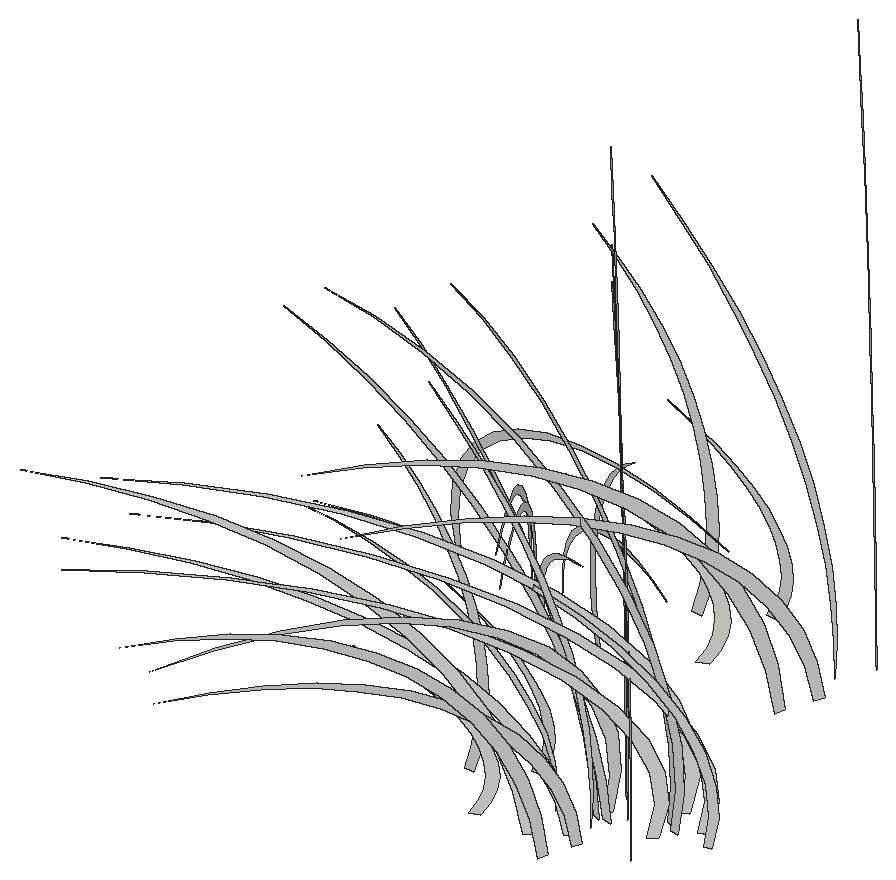
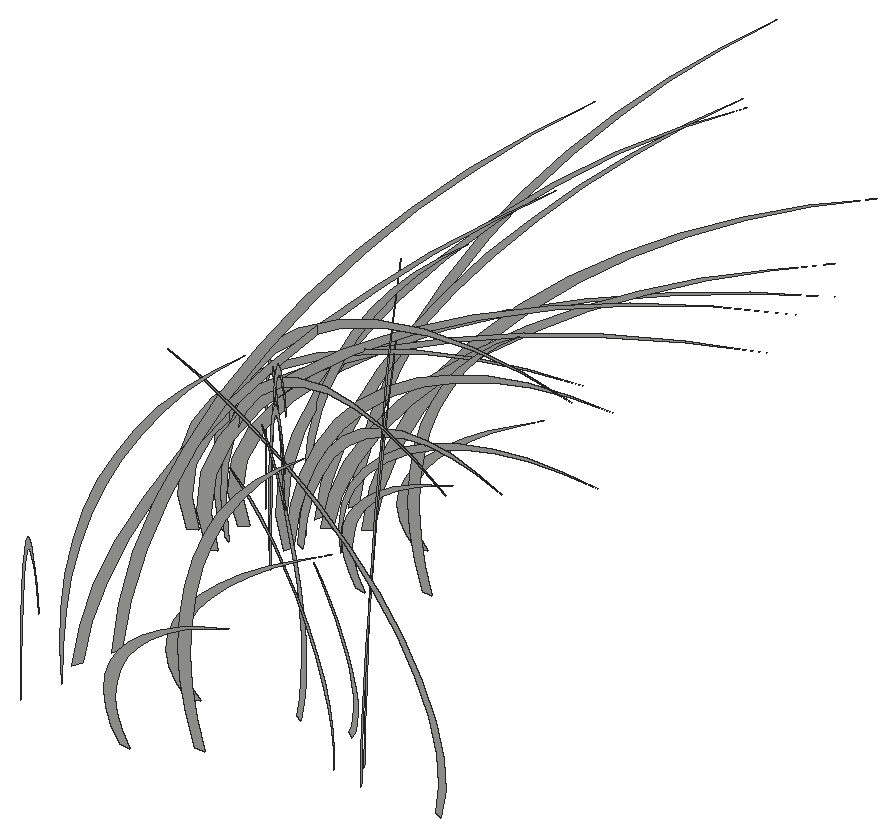
# SketchUp Ruby script. Lengths in inches.
U = 1.inch
M = Sketchup.active_model
def pt(a) = Geom::Point3d.new(a.map { |v| v * U })
def face(e, loops, mat)
  f = e.add_face(loops[0].map { |a| pt(a) })
  loops[1..].each { |l| e.add_face(l.map { |a| pt(a) }).erase! }
  f.material = f.back_material = mat if mat
  f
end
# faces: each face lists its corners as indices into pts; further lists are holes
def faces(e, pts, list, mat = nil) = list.each { |f| face(e, (f[0].is_a?(Array) ? f : [f]).map { |l| l.map { |i| pts[i] } }, mat) }
# xy, xz, yz: faces in a plane at the given z, y or x. An outline is a flat list of corners, or four numbers for a rectangle; further outlines are holes
def ring(l) = l.size == 4 ? [[l[0], l[1]], [l[2], l[1]], [l[2], l[3]], [l[0], l[3]]] : l.each_slice(2).to_a
def flat(e, list, mat, &to3) = list.each { |f| face(e, (f[0].is_a?(Array) ? f : [f]).map { |l| ring(l).map { |u, v| to3.(u, v) } }, mat) }
def xy(e, z, list, mat = nil) = flat(e, list, mat) { |x, y| [x, y, z] }
def xz(e, y, list, mat = nil) = flat(e, list, mat) { |x, z| [x, y, z] }
def yz(e, x, list, mat = nil) = flat(e, list, mat) { |y, z| [x, y, z] }
def lines(e, pts, list) = list.each { |a, b| e.add_line(pt(pts[a]), pt(pts[b])) }
# prism: a flat outline (further loops are holes) pulled along v
def prism(e, loops, v, mat = nil)
  f = face(e, loops, mat); d = Geom::Vector3d.new(v.map { |x| x * U })
  f.pushpull(f.normal.samedirection?(d) ? d.length : -d.length)
end
def box(e, o, s, mat = nil) = prism(e, [[o, [o[0] + s[0], o[1], o[2]], [o[0] + s[0], o[1] + s[1], o[2]], [o[0], o[1] + s[1], o[2]]]], [0, 0, s[2]], mat)
def at(x, y, z, deg = 0) = Geom::Transformation.translation(pt([x, y, z])) * Geom::Transformation.rotation(ORIGIN, Z_AXIS, deg.degrees)
def axes(o, x, y, z) = Geom::Transformation.new([*x, 0, *y, 0, *z, 0, *pt(o).to_a, 1])
def part(name) = M.definitions.add(name)
# library, detail: a bought-in or finely detailed component or shape, given as its bounding box
def library(name, o, s) = part(name).tap { |d| box(d.entities, o, s) }
def detail(e, o, s) = box(e.add_group.entities, o, s)
def put(e, d, t, mat = nil) = e.add_instance(d, t).tap { |i| i.material = mat if mat }
def group(e, t, mat = nil) = e.add_group.tap { |g| g.transformation = t; g.material = mat if mat }.entities
root = M.entities
g1 = group(root,at(18.37,764.86,-58.625))
p = [[3.01,-1.98,3.36],[2.46,-1.62,3.15],[1.96,-1.29,2.92],[1.52,-1,2.66],[1.15,-0.75,2.4],[0.83,-0.55,2.12],
  [0.59,-0.39,1.82],[0.41,-0.27,1.52],[0.3125,-0.21,1.22],[0.28,-0.1875,0.91],[0.33,-0.21,0.6],[0.44,-0.29,0.3],
  [0.63,-0.41,0],[0.39,-0.25,0],[0.18,-0.12,0.3],[0.05,-0.03,0.61],[0,0,0.93],[0.03,-0.02,1.24],
  [0.15,-0.1,1.55],[0.34,-0.22,1.85],[0.61,-0.4,2.15],[0.96,-0.63,2.43],[1.38,-0.91,2.69],[1.86,-1.23,2.94],
  [2.41,-1.58,3.16]]
faces(g1,p,[[0,1,2,3,4,5,6,7,8,9,10,11,12,13,14,15,16,17,18,19,20,21,22,23,24]])
g2 = group(root,at(25.21,756.14,-58.625))
p = [[-9.2,-6.42,9.74],[-10.59,-7.39,10],[-9.24,-6.45,9.69],[-7.94,-5.54,9.26],[-6.71,-4.68,8.71],[-5.54,-3.87,8.06],
  [-4.47,-3.12,7.3],[-3.49,-2.44,6.45],[-2.625,-1.83,5.52],[-1.88,-1.31,4.52],[-1.26,-0.88,3.45],[-0.78,-0.54,2.33],
  [-0.4375,-0.3,1.18],[-0.24,-0.17,0],[0,0,0],[-0.16,-0.11,1.21],[-0.48,-0.34,2.39],[-0.96,-0.67,3.53],
  [-1.58,-1.1,4.625],[-2.34,-1.63,5.65],[-3.23,-2.25,6.6],[-4.24,-2.96,7.45],[-5.36,-3.74,8.2],[-6.57,-4.58,8.84],
  [-7.85,-5.48,9.35]]
faces(g2,p,[[0,1,2,3,4,5,6,7,8,9,10,11,12,13,14,15,16,17,18,19,20,21,22,23,24]])
g3 = group(root,at(22.1,767.41,-58.625))
p = [[-4.36,0.43,9.78],[-3.5625,0.35,9.15],[-2.84,0.28,8.47],[-2.21,0.22,7.74],[-1.66,0.16,6.96],[-1.21,0.12,6.15],
  [-0.85,0.08,5.3],[-0.6,0.06,4.43],[-0.45,0.04,3.54],[-0.41,0.04,2.65],[-0.47,0.05,1.75],[-0.64,0.0625,0.87],
  [-0.91,0.09,0],[-0.5625,0.06,0],[-0.26,0.03,0.88],[-0.07,0.01,1.78],[0,0,2.6875],[-0.05,0,3.6],
  [-0.21,0.02,4.5],[-0.49,0.05,5.39],[-0.89,0.09,6.24],[-1.39,0.14,7.06],[-2,0.2,7.83],[-2.7,0.26,8.54],
  [-3.49,0.34,9.19]]
faces(g3,p,[[0,1,2,3,4,5,6,7,8,9,10,11,12,13,14,15,16,17,18,19,20,21,22,23,24]])
g4 = group(root,at(22.1,767.41,-58.625))
p = [[-4.36,0.43,9.78],[-3.5625,0.35,9.15],[-2.84,0.28,8.47],[-2.21,0.22,7.74],[-1.66,0.16,6.96],[-1.21,0.12,6.15],
  [-0.85,0.08,5.3],[-0.6,0.06,4.43],[-0.45,0.04,3.54],[-0.41,0.04,2.65],[-0.47,0.05,1.75],[-0.64,0.0625,0.87],
  [-0.91,0.09,0],[-0.5625,0.06,0],[-0.26,0.03,0.88],[-0.07,0.01,1.78],[0,0,2.6875],[-0.05,0,3.6],
  [-0.21,0.02,4.5],[-0.49,0.05,5.39],[-0.89,0.09,6.24],[-1.39,0.14,7.06],[-2,0.2,7.83],[-2.7,0.26,8.54],
  [-3.49,0.34,9.19]]
faces(g4,p,[[0,1,2,3,4,5,6,7,8,9,10,11,12,13,14,15,16,17,18,19,20,21,22,23,24]])
g5 = group(root,at(26.37,757.75,-58.625))
p = [[-10.97,2.33,9.03],[-12.625,2.68,9.27],[-11.02,2.34,8.98],[-9.47,2.01,8.58],[-8,1.7,8.08],[-6.61,1.41,7.47],
  [-5.33,1.13,6.77],[-4.16,0.88,5.98],[-3.13,0.67,5.12],[-2.24,0.48,4.1875],[-1.5,0.32,3.2],[-0.93,0.2,2.16],
  [-0.52,0.11,1.09],[-0.29,0.0625,0],[0,0,0],[-0.19,0.04,1.12],[-0.57,0.12,2.22],[-1.14,0.24,3.28],
  [-1.88,0.4,4.29],[-2.79,0.59,5.24],[-3.85,0.82,6.11],[-5.06,1.08,6.9],[-6.39,1.36,7.6],[-7.83,1.67,8.19],
  [-9.37,1.99,8.67]]
faces(g5,p,[[0,1,2,3,4,5,6,7,8,9,10,11,12,13,14,15,16,17,18,19,20,21,22,23,24]])
g6 = group(root,at(26.02,757.7,-58.625))
p = [[-9.9,5.27,7.86],[-11.4,6.06,8.07],[-9.95,5.29,7.82],[-8.55,4.55,7.47],[-7.22,3.84,7.03],[-5.97,3.17,6.5],
  [-4.81,2.56,5.89],[-3.76,2,5.21],[-2.83,1.5,4.45],[-2.02,1.08,3.64],[-1.36,0.72,2.78],[-0.84,0.45,1.88],
  [-0.47,0.25,0.95],[-0.26,0.14,0],[0,0,0],[-0.17,0.09,0.97],[-0.52,0.28,1.93],[-1.03,0.55,2.85],
  [-1.7,0.9,3.73],[-2.52,1.34,4.56],[-3.48,1.85,5.32],[-4.57,2.43,6.01],[-5.77,3.07,6.61],[-7.07,3.76,7.125],
  [-8.46,4.5,7.54]]
faces(g6,p,[[0,1,2,3,4,5,6,7,8,9,10,11,12,13,14,15,16,17,18,19,20,21,22,23,24]])
g7 = group(root,at(17.03,766.43,-58.625))
p = [[5.875,-8.62,6.21],[6.76,-9.92,6.375],[5.9,-8.66,6.18],[5.07,-7.44,5.9],[4.28,-6.28,5.56],[3.54,-5.19,5.14],
  [2.85,-4.1875,4.66],[2.23,-3.27,4.11],[1.68,-2.46,3.52],[1.2,-1.76,2.88],[0.81,-1.18,2.2],[0.5,-0.73,1.49],
  [0.28,-0.41,0.75],[0.15,-0.22,0],[0,0,0],[0.1,-0.15,0.77],[0.31,-0.45,1.52],[0.61,-0.9,2.25],
  [1.01,-1.48,2.95],[1.49,-2.19,3.6],[2.0625,-3.03,4.21],[2.71,-3.98,4.75],[3.42,-5.02,5.23],[4.2,-6.15,5.63],
  [5.02,-7.36,5.96]]
faces(g7,p,[[0,1,2,3,4,5,6,7,8,9,10,11,12,13,14,15,16,17,18,19,20,21,22,23,24]])
g8 = group(root,at(24.98,757.38,-58.625))
p = [[-9.02,0.88,5.34],[-7.8125,0.77,5.31],[-6.62,0.65,5.18],[-5.47,0.54,4.96],[-4.38,0.43,4.65],[-3.38,0.33,4.26],
  [-2.48,0.24,3.79],[-1.71,0.17,3.26],[-1.07,0.1,2.67],[-0.58,0.06,2.04],[-0.25,0.02,1.375],[-0.08,0.01,0.69],
  [-0.08,0.01,0],[0,0,0.7],[-0.11,0.01,1.41],[-0.4,0.04,2.09],[-0.86,0.08,2.75],[-1.5,0.15,3.35],
  [-2.28,0.22,3.9],[-3.2,0.3125,4.37],[-4.24,0.42,4.76],[-5.36,0.53,5.06],[-6.55,0.64,5.26],[-7.78,0.76,5.35]]
faces(g8,p,[[0,1,2,3,4,5,6,7,8,9,10,11,12,13,14,15,16,17,18,19,20,21,22,23]])
g9 = group(root,at(22.55,757.62,-58.625))
p = [[-3.86,0.38,8.65],[-3.15,0.31,8.1],[-2.51,0.25,7.5],[-1.95,0.19,6.85],[-1.47,0.14,6.16],[-1.07,0.1,5.44],
  [-0.75,0.07,4.6875],[-0.53,0.05,3.92],[-0.4,0.04,3.13],[-0.36,0.04,2.34],[-0.42,0.04,1.55],[-0.57,0.06,0.77],
  [-0.81,0.08,0],[-0.5,0.05,0],[-0.23,0.02,0.78],[-0.0625,0.01,1.57],[0,0,2.38],[-0.04,0,3.1875],
  [-0.1875,0.02,3.99],[-0.4375,0.04,4.77],[-0.79,0.08,5.52],[-1.23,0.12,6.25],[-1.77,0.17,6.93],[-2.39,0.23,7.5625],
  [-3.09,0.3,8.14]]
faces(g9,p,[[0,1,2,3,4,5,6,7,8,9,10,11,12,13,14,15,16,17,18,19,20,21,22,23,24]])
g10 = group(root,at(22.55,757.62,-58.625))
p = [[-3.86,0.38,8.65],[-3.15,0.31,8.1],[-2.51,0.25,7.5],[-1.95,0.19,6.85],[-1.47,0.14,6.16],[-1.07,0.1,5.44],
  [-0.75,0.07,4.6875],[-0.53,0.05,3.92],[-0.4,0.04,3.13],[-0.36,0.04,2.34],[-0.42,0.04,1.55],[-0.57,0.06,0.77],
  [-0.81,0.08,0],[-0.5,0.05,0],[-0.23,0.02,0.78],[-0.0625,0.01,1.57],[0,0,2.38],[-0.04,0,3.1875],
  [-0.1875,0.02,3.99],[-0.4375,0.04,4.77],[-0.79,0.08,5.52],[-1.23,0.12,6.25],[-1.77,0.17,6.93],[-2.39,0.23,7.5625],
  [-3.09,0.3,8.14]]
faces(g10,p,[[0,1,2,3,4,5,6,7,8,9,10,11,12,13,14,15,16,17,18,19,20,21,22,23,24]])
g11 = group(root,at(26.0625,756.74,-58.625))
p = [[-9.2,-6.42,7.86],[-10.59,-7.39,8.07],[-9.24,-6.45,7.82],[-7.94,-5.54,7.47],[-6.71,-4.68,7.03],[-5.54,-3.87,6.5],
  [-4.47,-3.12,5.89],[-3.49,-2.44,5.21],[-2.625,-1.83,4.45],[-1.88,-1.31,3.64],[-1.26,-0.88,2.78],[-0.78,-0.54,1.88],
  [-0.4375,-0.3,0.95],[-0.24,-0.17,0],[0,0,0],[-0.16,-0.11,0.97],[-0.48,-0.34,1.93],[-0.96,-0.67,2.85],
  [-1.58,-1.1,3.73],[-2.34,-1.63,4.56],[-3.23,-2.25,5.32],[-4.24,-2.96,6.01],[-5.36,-3.74,6.61],[-6.57,-4.58,7.125],
  [-7.85,-5.48,7.54]]
faces(g11,p,[[0,1,2,3,4,5,6,7,8,9,10,11,12,13,14,15,16,17,18,19,20,21,22,23,24]])
g12 = group(root,at(14.26,766.49,-58.625))
p = [[0.46,-0.1875,0],[0.21,-0.08,0],[0,0,0.88],[0.08,-0.03,1.76],[0.45,-0.18,2.63],[1.1,-0.44,3.46],
  [2.01,-0.81,4.23],[3.16,-1.27,4.92],[4.51,-1.8125,5.51],[6.05,-2.43,6],[7.72,-3.1,6.36],[9.49,-3.81,6.59],
  [11.3125,-4.55,6.6875],[13.14,-5.28,6.64],[11.35,-4.5625,6.65],[9.57,-3.85,6.53],[7.85,-3.16,6.28],[6.23,-2.5,5.9],
  [4.74,-1.91,5.41],[3.43,-1.38,4.82],[2.31,-0.93,4.14],[1.43,-0.57,3.39],[0.79,-0.32,2.58],[0.41,-0.16,1.73],
  [0.3,-0.12,0.86]]
faces(g12,p,[[0,1,2,3,4,5,6,7,8,9,10,11,12,13,14,15,16,17,18,19,20,21,22,23,24]])
g13 = group(root,at(17.57,765.63,-58.625))
p = [[5.875,-8.62,7.7],[6.76,-9.92,7.91],[5.9,-8.66,7.66],[5.07,-7.44,7.32],[4.28,-6.28,6.89],[3.54,-5.19,6.37],
  [2.85,-4.1875,5.77],[2.23,-3.27,5.1],[1.68,-2.46,4.37],[1.2,-1.76,3.57],[0.81,-1.18,2.73],[0.5,-0.73,1.84],
  [0.28,-0.41,0.93],[0.15,-0.22,0],[0,0,0],[0.1,-0.15,0.95],[0.31,-0.45,1.89],[0.61,-0.9,2.79],
  [1.01,-1.48,3.66],[1.49,-2.19,4.47],[2.0625,-3.03,5.21],[2.71,-3.98,5.89],[3.42,-5.02,6.48],[4.2,-6.15,6.99],
  [5.02,-7.36,7.39]]
faces(g13,p,[[0,1,2,3,4,5,6,7,8,9,10,11,12,13,14,15,16,17,18,19,20,21,22,23,24]])
g14 = group(root,at(27.83,759.49,-58.625))
p = [[-0.47,-0.26,0],[-0.21,-0.11,0],[0,0,1.09],[-0.08,-0.05,2.18],[-0.46,-0.25,3.25],[-1.12,-0.61,4.27],
  [-2.04,-1.12,5.22],[-3.21,-1.76,6.08],[-4.59,-2.51,6.8125],[-6.15,-3.37,7.41],[-7.85,-4.3,7.86],[-9.65,-5.28,8.15],
  [-11.5,-6.3,8.26],[-13.36,-7.32,8.21],[-11.54,-6.32,8.22],[-9.73,-5.33,8.07],[-7.98,-4.37,7.76],[-6.33,-3.47,7.29],
  [-4.82,-2.64,6.69],[-3.49,-1.91,5.96],[-2.35,-1.29,5.12],[-1.45,-0.79,4.1875],[-0.8,-0.4375,3.18],[-0.41,-0.23,2.14],
  [-0.3,-0.17,1.07]]
faces(g14,p,[[0,1,2,3,4,5,6,7,8,9,10,11,12,13,14,15,16,17,18,19,20,21,22,23,24]])
g15 = group(root,at(28.29,758.28,-58.625))
p = [[-0.49,0.1,0],[-0.22,0.05,0],[0,0,1.28],[-0.09,0.02,2.5625],[-0.48,0.1,3.82],[-1.16,0.25,5.03],
  [-2.12,0.45,6.15],[-3.33,0.71,7.15],[-4.77,1.01,8.02],[-6.39,1.36,8.72],[-8.15,1.73,9.25],[-10.02,2.13,9.58],
  [-11.95,2.54,9.72],[-13.88,2.95,9.66],[-11.98,2.55,9.67],[-10.1,2.15,9.49],[-8.29,1.76,9.125],[-6.58,1.4,8.58],
  [-5.01,1.06,7.87],[-3.62,0.77,7.01],[-2.44,0.52,6.02],[-1.51,0.32,4.92],[-0.83,0.18,3.75],[-0.43,0.09,2.51],
  [-0.32,0.07,1.26]]
faces(g15,p,[[0,1,2,3,4,5,6,7,8,9,10,11,12,13,14,15,16,17,18,19,20,21,22,23,24]])
g16 = group(root,at(19.92,765,-58.625))
p = [[3.01,-1.98,6.84],[2.46,-1.62,6.4],[1.96,-1.29,5.93],[1.52,-1,5.42],[1.15,-0.75,4.87],[0.83,-0.55,4.3],
  [0.59,-0.39,3.71],[0.41,-0.27,3.1],[0.3125,-0.21,2.48],[0.28,-0.1875,1.85],[0.33,-0.21,1.23],[0.44,-0.29,0.61],
  [0.63,-0.41,0],[0.39,-0.25,0],[0.18,-0.12,0.61],[0.05,-0.03,1.24],[0,0,1.88],[0.03,-0.02,2.52],
  [0.15,-0.1,3.15],[0.34,-0.22,3.77],[0.61,-0.4,4.37],[0.96,-0.63,4.9375],[1.38,-0.91,5.48],[1.86,-1.23,5.98],
  [2.41,-1.58,6.43]]
faces(g16,p,[[0,1,2,3,4,5,6,7,8,9,10,11,12,13,14,15,16,17,18,19,20,21,22,23,24]])
g17 = group(root,at(23.68,768.44,-58.625))
p = [[-4.36,0.43,4.81],[-3.5625,0.35,4.5],[-2.84,0.28,4.17],[-2.21,0.22,3.81],[-1.66,0.16,3.43],[-1.21,0.12,3.02],
  [-0.85,0.08,2.61],[-0.6,0.06,2.18],[-0.45,0.04,1.74],[-0.41,0.04,1.3],[-0.47,0.05,0.86],[-0.64,0.0625,0.43],
  [-0.91,0.09,0],[-0.5625,0.06,0],[-0.26,0.03,0.43],[-0.07,0.01,0.875],[0,0,1.32],[-0.05,0,1.77],
  [-0.21,0.02,2.22],[-0.49,0.05,2.65],[-0.89,0.09,3.07],[-1.39,0.14,3.47],[-2,0.2,3.85],[-2.7,0.26,4.2],
  [-3.49,0.34,4.52]]
faces(g17,p,[[0,1,2,3,4,5,6,7,8,9,10,11,12,13,14,15,16,17,18,19,20,21,22,23,24]])
g18 = group(root,at(18.02,766.25,-58.625))
p = [[7.05,-4.63,4.22],[6.1,-4.01,4.2],[5.17,-3.4,4.09],[4.27,-2.81,3.92],[3.42,-2.25,3.67],[2.64,-1.74,3.36],
  [1.9375,-1.27,3],[1.33,-0.88,2.57],[0.84,-0.55,2.11],[0.45,-0.3,1.61],[0.19,-0.13,1.09],[0.0625,-0.04,0.55],
  [0.0625,-0.04,0],[0,0,0.56],[0.08,-0.05,1.11],[0.31,-0.2,1.65],[0.67,-0.44,2.17],[1.17,-0.77,2.65],
  [1.78,-1.17,3.08],[2.5,-1.64,3.46],[3.31,-2.17,3.76],[4.1875,-2.75,4],[5.12,-3.36,4.16],[6.08,-4,4.23]]
faces(g18,p,[[0,1,2,3,4,5,6,7,8,9,10,11,12,13,14,15,16,17,18,19,20,21,22,23]])
g19 = group(root,at(27.86,758.49,-58.625))
p = [[-0.44,0.23,0],[-0.2,0.1,0],[0,0,1.11],[-0.08,0.04,2.23],[-0.43,0.23,3.33],[-1.05,0.56,4.375],
  [-1.91,1.02,5.35],[-3.01,1.6,6.22],[-4.3,2.29,6.97],[-5.76,3.06,7.59],[-7.36,3.91,8.05],[-9.05,4.81,8.34],
  [-10.78,5.73,8.46],[-12.53,6.66,8.4],[-10.82,5.75,8.41],[-9.12,4.85,8.26],[-7.48,3.98,7.9375],[-5.9375,3.16,7.47],
  [-4.52,2.4,6.85],[-3.27,1.74,6.1],[-2.21,1.17,5.24],[-1.36,0.72,4.28],[-0.75,0.4,3.26],[-0.39,0.21,2.1875],
  [-0.28,0.15,1.09]]
faces(g19,p,[[0,1,2,3,4,5,6,7,8,9,10,11,12,13,14,15,16,17,18,19,20,21,22,23,24]])
g20 = group(root,at(23.75,765.85,-58.625))
p = [[-4.1,-1.53,4.81],[-3.35,-1.25,4.5],[-2.68,-1,4.17],[-2.08,-0.77,3.81],[-1.5625,-0.58,3.43],[-1.14,-0.42,3.02],
  [-0.8,-0.3,2.61],[-0.57,-0.21,2.18],[-0.43,-0.16,1.74],[-0.39,-0.14,1.3],[-0.44,-0.17,0.86],[-0.6,-0.22,0.43],
  [-0.86,-0.32,0],[-0.53,-0.2,0],[-0.24,-0.09,0.43],[-0.07,-0.02,0.875],[0,0,1.32],[-0.05,-0.02,1.77],
  [-0.2,-0.07,2.22],[-0.47,-0.17,2.65],[-0.84,-0.3125,3.07],[-1.31,-0.49,3.47],[-1.88,-0.7,3.85],[-2.54,-0.95,4.2],
  [-3.29,-1.22,4.52]]
faces(g20,p,[[0,1,2,3,4,5,6,7,8,9,10,11,12,13,14,15,16,17,18,19,20,21,22,23,24]])
g21 = group(root,at(25.91,758.97,-58.625))
p = [[-7.28,8.53,11.2],[-8.38,9.82,11.5],[-7.32,8.57,11.14],[-6.29,7.37,10.64],[-5.3125,6.22,10.02],[-4.39,5.14,9.26],
  [-3.54,4.14,8.4],[-2.76,3.24,7.42],[-2.08,2.43,6.35],[-1.49,1.74,5.19],[-1,1.17,3.97],[-0.62,0.72,2.68],
  [-0.35,0.4,1.35],[-0.19,0.22,0],[0,0,0],[-0.13,0.15,1.39],[-0.38,0.45,2.75],[-0.76,0.89,4.0625],
  [-1.25,1.46,5.32],[-1.85,2.17,6.5],[-2.56,3,7.58],[-3.36,3.93,8.5625],[-4.24,4.97,9.42],[-5.2,6.09,10.16],
  [-6.22,7.28,10.75]]
faces(g21,p,[[0,1,2,3,4,5,6,7,8,9,10,11,12,13,14,15,16,17,18,19,20,21,22,23,24]])
g22 = group(root,at(27.97,758.07,-58.625))
p = [[-0.44,-0.31,0],[-0.2,-0.14,0],[0,0,0.95],[-0.08,-0.06,1.9],[-0.43,-0.3,2.83],[-1.05,-0.73,3.72],
  [-1.91,-1.33,4.55],[-3,-2.09,5.29],[-4.29,-2.99,5.93],[-5.75,-4.01,6.45],[-7.34,-5.12,6.84],[-9.02,-6.29,7.09],
  [-10.75,-7.5,7.1875],[-12.49,-8.72,7.14],[-10.79,-7.52,7.15],[-9.09,-6.34,7.02],[-7.46,-5.2,6.75],[-5.92,-4.13,6.35],
  [-4.51,-3.14,5.82],[-3.26,-2.27,5.18],[-2.2,-1.53,4.45],[-1.36,-0.95,3.64],[-0.75,-0.52,2.77],[-0.39,-0.27,1.86],
  [-0.28,-0.2,0.93]]
faces(g22,p,[[0,1,2,3,4,5,6,7,8,9,10,11,12,13,14,15,16,17,18,19,20,21,22,23,24]])
g23 = group(root,at(27.97,758.07,-58.625))
p = [[-0.44,-0.31,0],[-0.2,-0.14,0],[0,0,0.95],[-0.08,-0.06,1.9],[-0.43,-0.3,2.83],[-1.05,-0.73,3.72],
  [-1.91,-1.33,4.55],[-3,-2.09,5.29],[-4.29,-2.99,5.93],[-5.75,-4.01,6.45],[-7.34,-5.12,6.84],[-9.02,-6.29,7.09],
  [-10.75,-7.5,7.1875],[-12.49,-8.72,7.14],[-10.79,-7.52,7.15],[-9.09,-6.34,7.02],[-7.46,-5.2,6.75],[-5.92,-4.13,6.35],
  [-4.51,-3.14,5.82],[-3.26,-2.27,5.18],[-2.2,-1.53,4.45],[-1.36,-0.95,3.64],[-0.75,-0.52,2.77],[-0.39,-0.27,1.86],
  [-0.28,-0.2,0.93]]
faces(g23,p,[[0,1,2,3,4,5,6,7,8,9,10,11,12,13,14,15,16,17,18,19,20,21,22,23,24]])
g24 = group(root,at(26.66,768.05,-58.625))
p = [[-8.23,9.64,10.21],[-9.47,11.09,10.48],[-8.27,9.68,10.15],[-7.11,8.32,9.7],[-6,7.03,9.13],[-4.96,5.81,8.44],
  [-4,4.68,7.65],[-3.125,3.66,6.76],[-2.35,2.75,5.78],[-1.68,1.97,4.73],[-1.13,1.32,3.61],[-0.7,0.82,2.44],
  [-0.39,0.46,1.23],[-0.21,0.25,0],[0,0,0],[-0.14,0.17,1.26],[-0.43,0.51,2.5],[-0.86,1,3.7],
  [-1.41,1.65,4.85],[-2.09,2.45,5.92],[-2.89,3.39,6.91],[-3.8,4.45,7.8],[-4.8,5.62,8.59],[-5.88,6.88,9.26],
  [-7.03,8.23,9.8]]
faces(g24,p,[[0,1,2,3,4,5,6,7,8,9,10,11,12,13,14,15,16,17,18,19,20,21,22,23,24]])
g25 = group(root,at(28.88,758.95,-58.625))
p = [[-0.49,-0.22,0],[-0.22,-0.1,0],[0,0,0.95],[-0.09,-0.04,1.9],[-0.48,-0.22,2.83],[-1.16,-0.52,3.72],
  [-2.12,-0.96,4.55],[-3.33,-1.5,5.29],[-4.77,-2.15,5.93],[-6.39,-2.88,6.45],[-8.15,-3.68,6.84],[-10.02,-4.53,7.09],
  [-11.95,-5.4,7.1875],[-13.88,-6.27,7.14],[-11.99,-5.41,7.15],[-10.11,-4.5625,7.02],[-8.29,-3.74,6.75],[-6.58,-2.97,6.35],
  [-5.01,-2.26,5.82],[-3.62,-1.64,5.18],[-2.44,-1.1,4.45],[-1.51,-0.68,3.64],[-0.83,-0.375,2.77],[-0.43,-0.19,1.86],
  [-0.32,-0.14,0.93]]
faces(g25,p,[[0,1,2,3,4,5,6,7,8,9,10,11,12,13,14,15,16,17,18,19,20,21,22,23,24]])
g26 = group(root,at(23.95,758.53,-58.625))
p = [[-3.86,0.38,4.26],[-3.15,0.31,3.98],[-2.51,0.25,3.6875],[-1.95,0.19,3.37],[-1.47,0.14,3.03],[-1.07,0.1,2.68],
  [-0.75,0.07,2.31],[-0.53,0.05,1.93],[-0.4,0.04,1.54],[-0.36,0.04,1.15],[-0.42,0.04,0.76],[-0.57,0.06,0.38],
  [-0.81,0.08,0],[-0.5,0.05,0],[-0.23,0.02,0.38],[-0.0625,0.01,0.77],[0,0,1.17],[-0.04,0,1.57],
  [-0.1875,0.02,1.96],[-0.4375,0.04,2.35],[-0.79,0.08,2.72],[-1.23,0.12,3.07],[-1.77,0.17,3.41],[-2.39,0.23,3.72],
  [-3.09,0.3,4]]
faces(g26,p,[[0,1,2,3,4,5,6,7,8,9,10,11,12,13,14,15,16,17,18,19,20,21,22,23,24]])
g27 = group(root,at(24.01,756.24,-58.625))
p = [[-3.63,-1.35,4.26],[-2.97,-1.1,3.98],[-2.37,-0.88,3.6875],[-1.84,-0.68,3.37],[-1.38,-0.51,3.03],[-1.01,-0.375,2.68],
  [-0.71,-0.26,2.31],[-0.5,-0.1875,1.93],[-0.375,-0.14,1.54],[-0.34,-0.125,1.15],[-0.39,-0.15,0.76],[-0.53,-0.2,0.38],
  [-0.76,-0.28,0],[-0.47,-0.17,0],[-0.22,-0.08,0.38],[-0.06,-0.02,0.77],[0,0,1.17],[-0.04,-0.01,1.57],
  [-0.18,-0.07,1.96],[-0.41,-0.15,2.35],[-0.74,-0.28,2.72],[-1.16,-0.43,3.07],[-1.66,-0.62,3.41],[-2.25,-0.84,3.72],
  [-2.91,-1.08,4]]
faces(g27,p,[[0,1,2,3,4,5,6,7,8,9,10,11,12,13,14,15,16,17,18,19,20,21,22,23,24]])
g28 = group(root,at(26.59,758.18,-58.625))
p = [[-7.28,8.53,9.03],[-8.38,9.82,9.27],[-7.32,8.57,8.98],[-6.29,7.37,8.58],[-5.3125,6.22,8.08],[-4.39,5.14,7.47],
  [-3.54,4.14,6.77],[-2.76,3.24,5.98],[-2.08,2.43,5.12],[-1.49,1.74,4.1875],[-1,1.17,3.2],[-0.62,0.72,2.16],
  [-0.35,0.4,1.09],[-0.19,0.22,0],[0,0,0],[-0.13,0.15,1.12],[-0.38,0.45,2.22],[-0.76,0.89,3.28],
  [-1.25,1.46,4.29],[-1.85,2.17,5.24],[-2.56,3,6.11],[-3.36,3.93,6.9],[-4.24,4.97,7.6],[-5.2,6.09,8.19],
  [-6.22,7.28,8.67]]
faces(g28,p,[[0,1,2,3,4,5,6,7,8,9,10,11,12,13,14,15,16,17,18,19,20,21,22,23,24]])
g29 = group(root,at(26.22,767.01,-58.625))
p = [[-6.45,0.63,11.96],[-5.42,0.53,11.08],[-4.47,0.4375,10.17],[-3.62,0.35,9.23],[-2.85,0.28,8.26],[-2.17,0.21,7.28],
  [-1.58,0.16,6.27],[-1.09,0.11,5.25],[-0.69,0.07,4.21],[-0.39,0.04,3.17],[-0.19,0.02,2.12],[-0.09,0.01,1.06],
  [-0.08,0.01,0],[0,0,1.0625],[-0.03,0,2.13],[-0.18,0.02,3.19],[-0.4375,0.04,4.25],[-0.8125,0.08,5.29],
  [-1.3,0.13,6.32],[-1.9,0.1875,7.33],[-2.6,0.26,8.32],[-3.41,0.33,9.28],[-4.33,0.42,10.21],[-5.34,0.52,11.1]]
faces(g29,p,[[0,1,2,3,4,5,6,7,8,9,10,11,12,13,14,15,16,17,18,19,20,21,22,23]])
g30 = group(root,at(28.1,756.41,-58.625))
p = [[-0.35,0.41,0],[-0.15,0.18,0],[0,0,1.09],[-0.0625,0.07,2.18],[-0.34,0.4,3.25],[-0.83,0.97,4.27],
  [-1.51,1.77,5.22],[-2.375,2.78,6.08],[-3.4,3.98,6.8125],[-4.55,5.33,7.41],[-5.81,6.8,7.86],[-7.14,8.36,8.15],
  [-8.51,9.97,8.26],[-9.89,11.58,8.21],[-8.54,10,8.22],[-7.2,8.43,8.07],[-5.91,6.92,7.76],[-4.6875,5.49,7.29],
  [-3.57,4.18,6.69],[-2.58,3.02,5.96],[-1.74,2.04,5.12],[-1.07,1.26,4.1875],[-0.59,0.69,3.18],[-0.31,0.36,2.14],
  [-0.22,0.26,1.07]]
faces(g30,p,[[0,1,2,3,4,5,6,7,8,9,10,11,12,13,14,15,16,17,18,19,20,21,22,23,24]])
g31 = group(root,at(26.2,757.26,-58.625))
p = [[-5.71,0.56,10.59],[-4.8,0.47,9.81],[-3.96,0.39,9],[-3.2,0.3125,8.17],[-2.52,0.25,7.3125],[-1.92,0.1875,6.4375],
  [-1.4,0.14,5.55],[-0.96,0.09,4.65],[-0.61,0.06,3.73],[-0.35,0.03,2.8],[-0.17,0.02,1.87],[-0.08,0.01,0.9375],
  [-0.07,0.01,0],[0,0,0.94],[-0.03,0,1.88],[-0.16,0.02,2.82],[-0.39,0.04,3.76],[-0.72,0.07,4.68],
  [-1.15,0.11,5.59],[-1.68,0.16,6.49],[-2.3,0.23,7.36],[-3.02,0.3,8.21],[-3.83,0.375,9.03],[-4.73,0.46,9.83]]
faces(g31,p,[[0,1,2,3,4,5,6,7,8,9,10,11,12,13,14,15,16,17,18,19,20,21,22,23]])
g32 = group(root,at(26.2,757.26,-58.625))
p = [[-5.71,0.56,10.59],[-4.8,0.47,9.81],[-3.96,0.39,9],[-3.2,0.3125,8.17],[-2.52,0.25,7.3125],[-1.92,0.1875,6.4375],
  [-1.4,0.14,5.55],[-0.96,0.09,4.65],[-0.61,0.06,3.73],[-0.35,0.03,2.8],[-0.17,0.02,1.87],[-0.08,0.01,0.9375],
  [-0.07,0.01,0],[0,0,0.94],[-0.03,0,1.88],[-0.16,0.02,2.82],[-0.39,0.04,3.76],[-0.72,0.07,4.68],
  [-1.15,0.11,5.59],[-1.68,0.16,6.49],[-2.3,0.23,7.36],[-3.02,0.3,8.21],[-3.83,0.375,9.03],[-4.73,0.46,9.83]]
faces(g32,p,[[0,1,2,3,4,5,6,7,8,9,10,11,12,13,14,15,16,17,18,19,20,21,22,23]])
g33 = group(root,at(29.35,758.35,-58.625))
p = [[-0.4,-0.07,0],[-0.18,-0.03,0],[0,0,0.91],[-0.07,-0.01,1.82],[-0.4,-0.06,2.72],[-0.96,-0.16,3.57],
  [-1.75,-0.29,4.36],[-2.76,-0.45,5.08],[-3.94,-0.65,5.69],[-5.28,-0.87,6.19],[-6.74,-1.1,6.57],[-8.29,-1.36,6.8],
  [-9.88,-1.62,6.9],[-11.48,-1.88,6.86],[-9.91,-1.625,6.86],[-8.36,-1.37,6.74],[-6.86,-1.12,6.48],[-5.44,-0.89,6.09],
  [-4.14,-0.68,5.59],[-3,-0.49,4.98],[-2.02,-0.33,4.28],[-1.25,-0.2,3.5],[-0.6875,-0.11,2.66],[-0.36,-0.06,1.79],
  [-0.26,-0.04,0.89]]
faces(g33,p,[[0,1,2,3,4,5,6,7,8,9,10,11,12,13,14,15,16,17,18,19,20,21,22,23,24]])
g34 = group(root,at(26.17,765.01,-58.625))
p = [[-3.83,-12.08,11.01],[-4.41,-13.9,11.3],[-3.85,-12.14,10.95],[-3.31,-10.43,10.46],[-2.79,-8.81,9.85],[-2.31,-7.28,9.11],
  [-1.86,-5.87,8.25],[-1.45,-4.58,7.29],[-1.09,-3.45,6.24],[-0.78,-2.47,5.1],[-0.53,-1.66,3.9],[-0.32,-1.02,2.64],
  [-0.18,-0.57,1.33],[-0.1,-0.31,0],[0,0,0],[-0.07,-0.21,1.36],[-0.2,-0.63,2.7],[-0.4,-1.26,3.99],
  [-0.66,-2.07,5.23],[-0.97,-3.07,6.39],[-1.35,-4.24,7.45],[-1.77,-5.57,8.42],[-2.23,-7.04,9.27],[-2.74,-8.625,9.99],
  [-3.27,-10.3125,10.57]]
faces(g34,p,[[0,1,2,3,4,5,6,7,8,9,10,11,12,13,14,15,16,17,18,19,20,21,22,23,24]])
g35 = group(root,at(26.17,765.01,-58.625))
p = [[-3.83,-12.08,11.01],[-4.41,-13.9,11.3],[-3.85,-12.14,10.95],[-3.31,-10.43,10.46],[-2.79,-8.81,9.85],[-2.31,-7.28,9.11],
  [-1.86,-5.87,8.25],[-1.45,-4.58,7.29],[-1.09,-3.45,6.24],[-0.78,-2.47,5.1],[-0.53,-1.66,3.9],[-0.32,-1.02,2.64],
  [-0.18,-0.57,1.33],[-0.1,-0.31,0],[0,0,0],[-0.07,-0.21,1.36],[-0.2,-0.63,2.7],[-0.4,-1.26,3.99],
  [-0.66,-2.07,5.23],[-0.97,-3.07,6.39],[-1.35,-4.24,7.45],[-1.77,-5.57,8.42],[-2.23,-7.04,9.27],[-2.74,-8.625,9.99],
  [-3.27,-10.3125,10.57]]
faces(g35,p,[[0,1,2,3,4,5,6,7,8,9,10,11,12,13,14,15,16,17,18,19,20,21,22,23,24]])
g36 = group(root,at(26.13,758.45,-58.625))
p = [[-0.15,-0.48,0],[-0.07,-0.21,0],[0,0,1.11],[-0.03,-0.09,2.23],[-0.15,-0.47,3.33],[-0.36,-1.13,4.375],
  [-0.66,-2.07,5.35],[-1.03,-3.25,6.22],[-1.47,-4.64,6.97],[-1.97,-6.22,7.59],[-2.52,-7.94,8.05],[-3.1,-9.77,8.34],
  [-3.69,-11.64,8.46],[-4.29,-13.53,8.4],[-3.7,-11.68,8.41],[-3.125,-9.85,8.26],[-2.5625,-8.08,7.9375],[-2.03,-6.41,7.47],
  [-1.55,-4.88,6.85],[-1.12,-3.53,6.1],[-0.76,-2.38,5.24],[-0.47,-1.47,4.28],[-0.26,-0.81,3.26],[-0.13,-0.42,2.1875],
  [-0.1,-0.31,1.09]]
faces(g36,p,[[0,1,2,3,4,5,6,7,8,9,10,11,12,13,14,15,16,17,18,19,20,21,22,23,24]])
g37 = group(root,at(26.16,755.49,-58.625))
p = [[-3.39,-10.69,9.74],[-3.9,-12.3,10],[-3.41,-10.74,9.69],[-2.93,-9.23,9.26],[-2.47,-7.79,8.71],[-2.04,-6.44,8.06],
  [-1.65,-5.19,7.3],[-1.29,-4.06,6.45],[-0.97,-3.05,5.52],[-0.69,-2.18,4.52],[-0.46,-1.47,3.45],[-0.29,-0.9,2.33],
  [-0.16,-0.51,1.18],[-0.09,-0.28,0],[0,0,0],[-0.06,-0.1875,1.21],[-0.18,-0.56,2.39],[-0.35,-1.11,3.53],
  [-0.58,-1.83,4.625],[-0.86,-2.72,5.65],[-1.19,-3.76,6.6],[-1.5625,-4.93,7.45],[-1.98,-6.23,8.2],[-2.42,-7.63,8.84],
  [-2.9,-9.13,9.35]]
faces(g37,p,[[0,1,2,3,4,5,6,7,8,9,10,11,12,13,14,15,16,17,18,19,20,21,22,23,24]])
g38 = group(root,at(26.16,755.49,-58.625))
p = [[-3.39,-10.69,9.74],[-3.9,-12.3,10],[-3.41,-10.74,9.69],[-2.93,-9.23,9.26],[-2.47,-7.79,8.71],[-2.04,-6.44,8.06],
  [-1.65,-5.19,7.3],[-1.29,-4.06,6.45],[-0.97,-3.05,5.52],[-0.69,-2.18,4.52],[-0.46,-1.47,3.45],[-0.29,-0.9,2.33],
  [-0.16,-0.51,1.18],[-0.09,-0.28,0],[0,0,0],[-0.06,-0.1875,1.21],[-0.18,-0.56,2.39],[-0.35,-1.11,3.53],
  [-0.58,-1.83,4.625],[-0.86,-2.72,5.65],[-1.19,-3.76,6.6],[-1.5625,-4.93,7.45],[-1.98,-6.23,8.2],[-2.42,-7.63,8.84],
  [-2.9,-9.13,9.35]]
faces(g38,p,[[0,1,2,3,4,5,6,7,8,9,10,11,12,13,14,15,16,17,18,19,20,21,22,23,24]])
g39 = group(root,at(26.53,766.13,-58.625))
p = [[-3.83,-12.08,8.88],[-4.41,-13.9,9.11],[-3.85,-12.14,8.83],[-3.31,-10.43,8.4375],[-2.79,-8.81,7.94],[-2.31,-7.28,7.34],
  [-1.86,-5.87,6.66],[-1.45,-4.58,5.88],[-1.09,-3.45,5.03],[-0.78,-2.47,4.12],[-0.53,-1.66,3.14],[-0.32,-1.02,2.125],
  [-0.18,-0.57,1.07],[-0.1,-0.31,0],[0,0,0],[-0.07,-0.21,1.1],[-0.2,-0.63,2.18],[-0.4,-1.26,3.22],
  [-0.66,-2.07,4.22],[-0.97,-3.07,5.15],[-1.35,-4.24,6.01],[-1.77,-5.57,6.79],[-2.23,-7.04,7.47],[-2.74,-8.625,8.05],
  [-3.27,-10.3125,8.52]]
faces(g39,p,[[0,1,2,3,4,5,6,7,8,9,10,11,12,13,14,15,16,17,18,19,20,21,22,23,24]])
g40 = group(root,at(26.47,756.48,-58.625))
p = [[-3.39,-10.69,7.86],[-3.9,-12.3,8.07],[-3.41,-10.74,7.82],[-2.93,-9.23,7.47],[-2.47,-7.79,7.03],[-2.04,-6.44,6.5],
  [-1.65,-5.19,5.89],[-1.29,-4.06,5.21],[-0.97,-3.05,4.45],[-0.69,-2.18,3.64],[-0.46,-1.47,2.78],[-0.29,-0.9,1.88],
  [-0.16,-0.51,0.95],[-0.09,-0.28,0],[0,0,0],[-0.06,-0.1875,0.97],[-0.18,-0.56,1.93],[-0.35,-1.11,2.85],
  [-0.58,-1.83,3.73],[-0.86,-2.72,4.56],[-1.19,-3.76,5.32],[-1.5625,-4.93,6.01],[-1.98,-6.23,6.61],[-2.42,-7.63,7.125],
  [-2.9,-9.13,7.54]]
faces(g40,p,[[0,1,2,3,4,5,6,7,8,9,10,11,12,13,14,15,16,17,18,19,20,21,22,23,24]])
g41 = group(root,at(26.47,756.48,-58.625))
p = [[-3.39,-10.69,7.86],[-3.9,-12.3,8.07],[-3.41,-10.74,7.82],[-2.93,-9.23,7.47],[-2.47,-7.79,7.03],[-2.04,-6.44,6.5],
  [-1.65,-5.19,5.89],[-1.29,-4.06,5.21],[-0.97,-3.05,4.45],[-0.69,-2.18,3.64],[-0.46,-1.47,2.78],[-0.29,-0.9,1.88],
  [-0.16,-0.51,0.95],[-0.09,-0.28,0],[0,0,0],[-0.06,-0.1875,0.97],[-0.18,-0.56,1.93],[-0.35,-1.11,2.85],
  [-0.58,-1.83,3.73],[-0.86,-2.72,4.56],[-1.19,-3.76,5.32],[-1.5625,-4.93,6.01],[-1.98,-6.23,6.61],[-2.42,-7.63,7.125],
  [-2.9,-9.13,7.54]]
faces(g41,p,[[0,1,2,3,4,5,6,7,8,9,10,11,12,13,14,15,16,17,18,19,20,21,22,23,24]])
